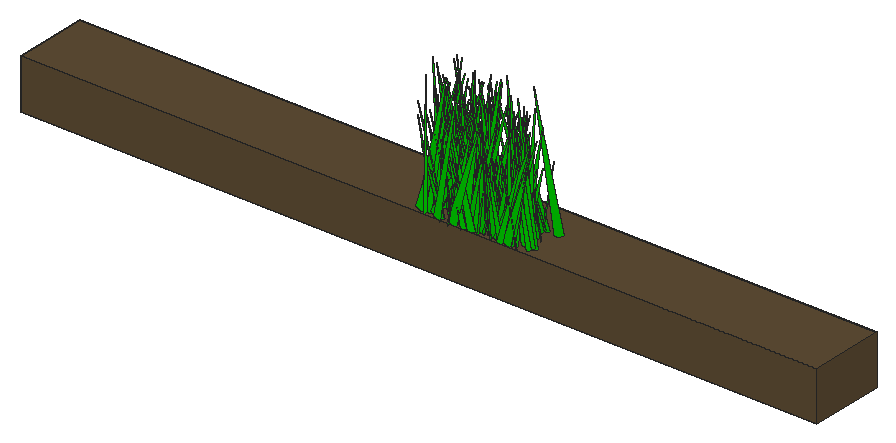
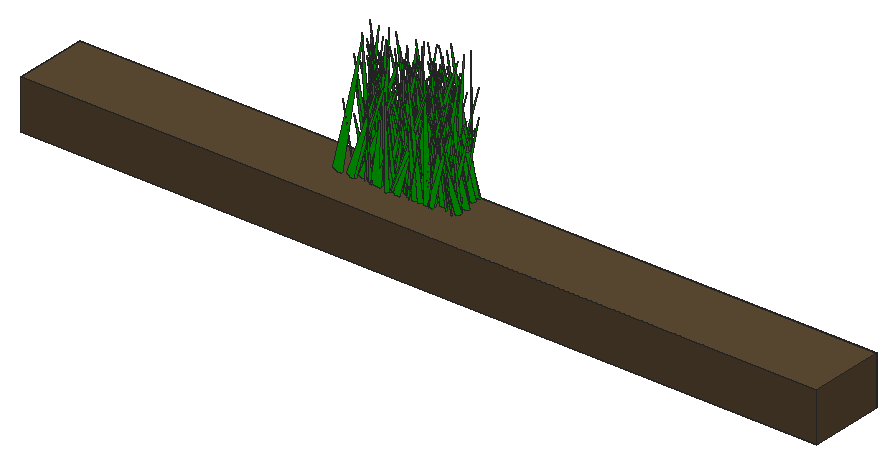
# SketchUp Ruby script. Lengths in inches.
U = 1.inch
M = Sketchup.active_model
def pt(a) = Geom::Point3d.new(a.map { |v| v * U })
def face(e, loops, mat)
  f = e.add_face(loops[0].map { |a| pt(a) })
  loops[1..].each { |l| e.add_face(l.map { |a| pt(a) }).erase! }
  f.material = f.back_material = mat if mat
  f
end
# faces: each face lists its corners as indices into pts; further lists are holes
def faces(e, pts, list, mat = nil) = list.each { |f| face(e, (f[0].is_a?(Array) ? f : [f]).map { |l| l.map { |i| pts[i] } }, mat) }
# xy, xz, yz: faces in a plane at the given z, y or x. An outline is a flat list of corners, or four numbers for a rectangle; further outlines are holes
def ring(l) = l.size == 4 ? [[l[0], l[1]], [l[2], l[1]], [l[2], l[3]], [l[0], l[3]]] : l.each_slice(2).to_a
def flat(e, list, mat, &to3) = list.each { |f| face(e, (f[0].is_a?(Array) ? f : [f]).map { |l| ring(l).map { |u, v| to3.(u, v) } }, mat) }
def xy(e, z, list, mat = nil) = flat(e, list, mat) { |x, y| [x, y, z] }
def xz(e, y, list, mat = nil) = flat(e, list, mat) { |x, z| [x, y, z] }
def yz(e, x, list, mat = nil) = flat(e, list, mat) { |y, z| [x, y, z] }
def lines(e, pts, list) = list.each { |a, b| e.add_line(pt(pts[a]), pt(pts[b])) }
# prism: a flat outline (further loops are holes) pulled along v
def prism(e, loops, v, mat = nil)
  f = face(e, loops, mat); d = Geom::Vector3d.new(v.map { |x| x * U })
  f.pushpull(f.normal.samedirection?(d) ? d.length : -d.length)
end
def box(e, o, s, mat = nil) = prism(e, [[o, [o[0] + s[0], o[1], o[2]], [o[0] + s[0], o[1] + s[1], o[2]], [o[0], o[1] + s[1], o[2]]]], [0, 0, s[2]], mat)
def at(x, y, z, deg = 0) = Geom::Transformation.translation(pt([x, y, z])) * Geom::Transformation.rotation(ORIGIN, Z_AXIS, deg.degrees)
def axes(o, x, y, z) = Geom::Transformation.new([*x, 0, *y, 0, *z, 0, *pt(o).to_a, 1])
def part(name) = M.definitions.add(name)
# library, detail: a bought-in or finely detailed component or shape, given as its bounding box
def library(name, o, s) = part(name).tap { |d| box(d.entities, o, s) }
def detail(e, o, s) = box(e.add_group.entities, o, s)
def put(e, d, t, mat = nil) = e.add_instance(d, t).tap { |i| i.material = mat if mat }
def group(e, t, mat = nil) = e.add_group.tap { |g| g.transformation = t; g.material = mat if mat }.entities
root = M.entities
M.materials.add("SOIL").color = [94, 77, 53]
M.materials.add("[Color G06]").color = [0, 204, 0]
c1 = part("fur_instance\#9")
p = [[0.8125,0,1.79],[0.67,-0.02,1.48],[0,-0.11,0],[0,0.11,0]]
faces(c1.entities,p,[[0,1,2,3]])
c2 = part("SOIL")
box(c2.entities,[0,0,0],[23.62,15.75,0.98],"SOIL")
put(root,c1,axes([64.27,19.94,4.28],[3.9337,-0.10201,2.1744],[-1.23525,-0.53254,2.12165],[-1.06111,0.24176,5.59098]),"[Color G06]")
put(root,c1,axes([66.12,17.16,4.28],[-3.59568,-0.13871,1.08691],[-1.16064,0.48631,-1.44733],[0.41383,0.15871,5.38474]),"[Color G06]")
put(root,c1,axes([66.23,19.01,4.28],[-2.06778,0.38398,1.15766],[2.83464,0.2572,1.51011],[-0.3835,-0.16929,4.92009]),"[Color G06]")
put(root,c1,axes([65.64,18.91,4.28],[-2.34714,-0.24884,0.13469],[-1.68843,0.31567,1.2736],[0.58467,-0.08736,4.21868]),"[Color G06]")
put(root,c2,axes([12.21,15.88,-2.33],[4.48996,0,0],[0,0.6261,0],[0,0,6.71057]),"[Color G06]")
put(root,c1,axes([65.53,16.66,4.28],[-4.03008,-0.15258,2.55922],[-0.6332,0.59823,1.86996],[1.93093,-0.12229,5.9546]),"[Color G06]")
put(root,c1,axes([64.93,20.74,4.28],[5.56804,0.19263,1.94531],[1.18681,-0.79236,1.42534],[-1.48118,0.08926,8.45483]),"[Color G06]")
put(root,c1,axes([65.28,18.91,4.28],[-4.27988,-0.612,0.13864],[-3.47082,0.48283,5.50199],[2.68766,-0.35103,7.32598]),"[Color G06]")
put(root,c1,axes([66.875,19.08,4.28],[0.00173,-0.4781,0.37924],[-3.2834,-0.01072,-1.51908],[-1.0193,0.03372,4.89395]),"[Color G06]")
put(root,c1,axes([64.82,18.02,4.28],[4.41749,0.02868,0.97094],[-0.02479,-0.58705,2.24414],[-0.68098,0.20744,6.21676]),"[Color G06]")
put(root,c1,axes([66.66,18.07,4.28],[2.23144,-0.72846,3.30583],[-5.41989,-0.37165,-1.23578],[-1.6756,0.23202,8.39972]),"[Color G06]")
put(root,c1,axes([66.01,18.3,4.28],[2.74843,0.58472,1.17107],[4.10613,-0.39786,1.29411],[-1.15604,-0.02302,7.38067]),"[Color G06]")
put(root,c1,axes([65.93,16.13,4.28],[5.28818,-0.28174,2.69175],[-1.63303,-0.7717,-2.11244],[-2.15849,-0.10641,8.19284]),"[Color G06]")
put(root,c1,axes([67.66,19.3,4.28],[-4.5157,0.45036,1.85261],[3.42037,0.6238,1.20327],[0.5177,-0.19305,8.2098]),"[Color G06]")
put(root,c1,axes([64.86,18.26,4.28],[1.2715,-0.352,0.82952],[-2.32783,-0.11849,2.1945],[1.12305,0.15293,3.60956]),"[Color G06]")
put(root,c1,axes([64.29,20.21,4.28],[2.89965,-0.47126,0.48649],[-3.21633,-0.36216,2.52086],[1.08732,0.18544,6.15941]),"[Color G06]")
put(root,c1,axes([67.61,20.84,4.28],[0.74196,-0.52967,0.07225],[-3.46204,-0.09711,-2.36776],[-1.56343,-0.03632,5.27742]),"[Color G06]")
put(root,c1,axes([65.63,18.85,4.28],[1.34326,0.36408,0.84996],[2.64038,-0.1672,-1.09373],[0.41087,-0.11584,4.24991]),"[Color G06]")
put(root,c1,axes([68.07,16.52,4.28],[-4.76111,-0.23036,0.10058],[-1.58818,0.64517,1.81412],[0.45963,-0.15694,7.31027]),"[Color G06]")
put(root,c1,axes([64.39,18.875,4.28],[3.81948,0.65894,0.41305],[4.68317,-0.51885,-1.64937],[0.68832,-0.12631,8.93]),"[Color G06]")
put(root,c1,axes([66.84,17.08,4.28],[-3.36168,0.48783,1.26493],[3.33459,0.4829,-1.59837],[1.35477,0.02188,7.07294]),"[Color G06]")
put(root,c1,axes([65.9,18.96,4.28],[-4.17835,0.54975,0.89849],[2.79534,0.49034,-5.42673],[2.84426,0.3257,6.65331]),"[Color G06]")
put(root,c1,axes([67.83,20.375,4.28],[-0.79878,-0.71008,0.86951],[-5.06087,0.0963,-1.35143],[-0.81022,0.09857,7.58425]),"[Color G06]")
put(root,c1,axes([68.07,16.24,4.28],[-1.79719,-0.34848,0.05868],[-2.42683,0.24169,-1.14114],[-0.59772,0.06647,4.45677]),"[Color G06]")
put(root,c1,axes([64.9375,16.33,4.28],[2.13707,0.68454,1.01733],[4.81023,-0.26161,-2.34953],[1.19326,-0.1714,7.64932]),"[Color G06]")
put(root,c1,axes([65.19,16.55,4.28],[-1.2259,-0.82669,2.42771],[-5.62709,0.24389,3.1931],[2.47397,0.14508,8.46575]),"[Color G06]")
put(root,c1,axes([66.25,18.01,4.28],[3.08494,0.15001,0.2605],[0.88845,-0.38846,2.19393],[-0.63105,0.18641,4.36231]),"[Color G06]")
put(root,c1,axes([66.37,19.62,4.28],[-1.44395,0.338,1.23713],[2.15076,0.23196,-1.67262],[1.39086,-0.00779,3.87082]),"[Color G06]")
put(root,c1,axes([65.86,20.33,4.28],[5.05978,0.1564,1.77856],[1.34323,-0.70526,-1.41146],[-0.93265,-0.16723,7.61609]),"[Color G06]")
put(root,c1,axes([64.8125,17.16,4.28],[5.71437,-0.35675,0.81278],[-2.61535,-0.7814,1.67358],[-0.02906,0.17354,9.20654]),"[Color G06]")
put(root,c1,axes([66.28,19.2,4.28],[4.30909,-0.14199,2.05065],[-1.42182,-0.58584,2.01409],[-0.94751,0.23337,6.30366]),"[Color G06]")
put(root,c1,axes([69.3125,19.57,4.28],[-5.52745,0.03843,0.24282],[0.22598,0.74656,-2.08225],[0.22645,0.19303,8.00506]),"[Color G06]")
put(root,c1,axes([67.84,20.68,4.28],[-3.57294,0.06411,1.38728],[0.20503,0.49942,-1.47175],[1.01534,0.12475,5.17899]),"[Color G06]")
put(root,c1,axes([66.63,19.9,4.28],[-1.10752,-0.6635,1.1429],[-4.62289,0.17718,1.80941],[1.36144,0.06188,7.07373]),"[Color G06]")
put(root,c1,axes([67.22,18.42,4.28],[4.87658,0.467,1.34273],[2.8491,-0.66289,3.37128],[-1.97624,0.1967,8.17365]),"[Color G06]")
put(root,c1,axes([66.07,16.44,4.28],[4.96611,-0.36753,1.97979],[-2.87532,-0.6839,1.52607],[-0.65883,0.21437,8.26304]),"[Color G06]")
put(root,c1,axes([66.57,17.35,4.28],[-0.59285,0.44163,1.9606],[3.16914,0.14138,-1.51769],[1.30675,-0.14251,4.57019]),"[Color G06]")
put(root,c1,axes([68.84,17.19,4.28],[-4.91803,-0.20416,0.17663],[-1.24803,0.61118,3.52939],[0.77451,-0.31152,6.80875]),"[Color G06]")
put(root,c1,axes([68.7,20.35,4.28],[-5.8108,0.01733,2.20475],[-0.05639,0.83002,-1.08167],[1.47933,0.09973,8.61904]),"[Color G06]")
put(root,c1,axes([68,17.33,4.28],[-2.34423,-0.18821,0.49656],[-1.15107,0.31378,1.5235],[0.77914,-0.1027,3.74478]),"[Color G06]")
put(root,c1,axes([69.53,20.3,4.28],[-2.66158,0.52184,0.92971],[3.72924,0.34047,1.89447],[-0.69586,-0.17132,6.59678]),"[Color G06]")
put(root,c1,axes([66.15,18.34,4.28],[4.53169,0.0066,0.17546],[0.00744,-0.59921,2.15905],[-0.12635,0.20134,6.41998]),"[Color G06]")
put(root,c1,axes([69.43,16.26,4.28],[-5.68691,0.08802,1.10084],[0.3155,0.74548,-3.20639],[0.91727,0.28928,7.92784]),"[Color G06]")
put(root,c1,axes([70.48,17.39,4.28],[-1.74227,-0.51191,0.57615],[-3.12279,0.17272,-3.46489],[-1.96806,0.17912,4.98781]),"[Color G06]")
put(root,c1,axes([65.21,19.46,4.28],[5.78095,-0.27577,0.1135],[-1.90726,-0.76757,2.75583],[0.52838,0.24657,8.70587]),"[Color G06]")
put(root,c1,axes([67.34,16.21,4.28],[-0.97561,0.32933,1.80319],[2.35163,0.1903,-1.15043],[1.22598,-0.10295,3.64164]),"[Color G06]")
put(root,c1,axes([67.75,19.18,4.28],[3.09749,-0.22392,0.88391],[-1.41414,-0.43098,-1.47269],[-0.96366,-0.08731,5.00229]),"[Color G06]")
put(root,c1,axes([68,19.7,4.28],[2.92193,-0.21443,1.09605],[-1.31963,-0.41328,-1.42956],[-1.07745,-0.07533,4.72326]),"[Color G06]")
put(root,c1,axes([66.02,17.58,4.28],[2.45604,-0.70792,0.71225],[-4.85278,-0.30188,2.91186],[1.56531,0.17488,7.90979]),"[Color G06]")
put(root,c1,axes([68,20.78,4.28],[-1.27431,-0.73556,1.5677],[-5.26886,0.20089,1.26122],[1.07877,0.1123,8.01183]),"[Color G06]")
put(root,c1,axes([65.85,19.25,4.28],[3.02053,-0.58933,0.27626],[-3.90663,-0.37645,3.15948],[1.62277,0.19067,7.09185]),"[Color G06]")
put(root,c1,axes([68.76,18.32,4.28],[3.35805,0.30855,1.56651],[1.83431,-0.48137,2.10828],[-1.62168,0.09443,5.62853]),"[Color G06]")
put(root,c1,axes([66.32,18.14,4.28],[5.01438,0.22789,0.47335],[1.61835,-0.63452,-3.20234],[0.39,-0.29709,7.20253]),"[Color G06]")
put(root,c1,axes([70.48,19.6,4.28],[-3.13704,-0.74976,1.17592],[-5.41814,0.42191,-1.38487],[-0.41462,0.15934,9.20002]),"[Color G06]")
put(root,c1,axes([67.78,19.27,4.28],[-1.94172,-0.3878,3.30736],[-2.88964,0.37698,1.28819],[2.06906,0.16255,4.90289]),"[Color G06]")
put(root,c1,axes([67.59,15.91,4.28],[3.54088,0.51335,2.57501],[4.06154,-0.45916,-1.96012],[-0.15678,-0.30115,7.37812]),"[Color G06]")
put(root,c1,axes([69.05,17.05,4.28],[-3.17062,0.45416,0.91994],[3.06388,0.4469,-1.7563],[1.26446,0.05594,6.5624]),"[Color G06]")
put(root,c1,axes([68.75,17.77,4.28],[4.24094,-0.29055,3.7921],[-2.78852,-0.62384,1.47521],[-1.73297,0.29279,6.90627]),"[Color G06]")
put(root,c1,axes([71.55,17.78,4.28],[-5.17247,-0.46056,0.00062],[-3.27844,0.71595,-1.11271],[-0.40033,0.08753,9.10447]),"[Color G06]")
put(root,c1,axes([68.38,18.43,4.28],[-1.87229,-0.7605,1.04521],[-5.23346,0.27808,2.30206],[1.68632,0.01863,8.30486]),"[Color G06]")
put(root,c1,axes([66.77,16.4,4.28],[2.33579,0.49121,0.1582],[3.08444,-0.27637,-3.14717],[1.7048,-0.17299,5.47731]),"[Color G06]")
put(root,c1,axes([69.96,17.8,4.28],[0.9333,-0.63025,1.21187],[-4.43375,-0.1537,-1.55525],[-1.19446,0.07809,6.71987]),"[Color G06]")
put(root,c1,axes([68.34,19.38,4.28],[3.11376,0.25616,0.9973],[1.94448,-0.42367,-1.06016],[-0.19703,-0.13299,5.29824]),"[Color G06]")
put(root,c1,axes([68.78,19.79,4.28],[-1.77394,0.70053,1.87694],[4.92633,0.28534,-1.83386],[1.59562,-0.10216,7.74859]),"[Color G06]")
put(root,c1,axes([68.23,18.93,4.28],[0.76642,0.55479,0.85726],[3.87739,-0.08056,-1.75415],[1.06014,-0.10644,5.79597]),"[Color G06]")
put(root,c1,axes([68.67,18.69,4.28],[0.09815,0.48947,2.17089],[3.68366,0.03723,-1.33642],[0.92802,-0.19956,5.07514]),"[Color G06]")
put(root,c1,axes([70.64,17.76,4.28],[-2.64218,-0.5957,2.25383],[-4.53026,0.34741,-1.31518],[-0.00041,0.24347,7.3911]),"[Color G06]")
put(root,c1,axes([68.59,18.15,4.28],[-0.66244,0.63721,1.68644],[4.49181,0.13307,-1.83449],[1.40654,-0.12484,6.65274]),"[Color G06]")
put(root,c1,axes([70.63,20.5625,4.28],[-3.75467,0.03192,0.77655],[0.07252,0.50757,-1.61376],[0.56313,0.14749,5.38546]),"[Color G06]")
put(root,c1,axes([69.33,15.95,4.28],[3.14663,0.29996,0.76242],[1.92015,-0.43215,1.82907],[-1.09564,0.10412,5.39514]),"[Color G06]")
put(root,c1,axes([68.43,18.98,4.28],[3.89803,-0.05532,0.69047],[-0.52017,-0.51951,1.7781],[-0.31662,0.1724,5.57952]),"[Color G06]")
put(root,c1,axes([70.31,19.58,4.28],[-3.14948,-0.17379,0.85258],[-0.96371,0.42253,1.94177],[0.97463,-0.1438,4.67506]),"[Color G06]")
put(root,c1,axes([71.11,15.96,4.28],[-2.60426,0.31734,0.66766],[2.31494,0.35007,1.05631],[-0.13964,-0.11495,5.05986]),"[Color G06]")
put(root,c1,axes([69,20.73,4.28],[4.80759,-0.32738,2.5492],[-2.66959,-0.67939,1.22332],[-1.13763,0.21079,7.90214]),"[Color G06]")
put(root,c1,axes([68.38,19.17,4.28],[4.77946,-0.11552,0.35589],[-0.76083,-0.65332,-1.53635],[-0.40506,-0.13587,7.0851]),"[Color G06]")
put(root,c1,axes([68.74,18.33,4.28],[3.73699,0.09804,0.06654],[0.64732,-0.49107,1.91444],[-0.27806,0.17447,5.35104]),"[Color G06]")
put(root,c1,axes([69.74,20.74,4.28],[-0.83593,0.48498,0.0355],[3.40191,0.11472,-1.10362],[0.72342,0.02091,5.23086]),"[Color G06]")
put(root,c1,axes([72.08,16.22,4.28],[-2.79763,-0.54176,1.73604],[-3.93774,0.31597,-2.84743],[-0.9682,0.28033,6.56439]),"[Color G06]")
put(root,c1,axes([70.22,17.8,4.28],[3.52732,0.2393,1.90503],[1.22279,-0.50717,2.26093],[-1.75339,0.12771,5.40912]),"[Color G06]")
put(root,c1,axes([68.68,18.1875,4.28],[-0.38735,-0.50805,1.24588],[-3.30073,0.10132,2.45407],[1.7533,0.07851,4.89525]),"[Color G06]")
put(root,c1,axes([72.33,20.92,4.28],[-0.69251,-0.73769,0.90073],[-4.94749,0.05784,-3.05542],[-1.96768,0.11421,7.36545]),"[Color G06]")
put(root,c1,axes([71.04,20.35,4.28],[-4.47876,0.12906,1.72291],[0.69894,0.63677,-1.42098],[1.30269,0.10208,6.68593]),"[Color G06]")
put(root,c1,axes([72.41,20.88,4.28],[-4.00422,0.36649,1.21006],[2.71666,0.49613,2.81914],[-0.42755,-0.27996,6.58009]),"[Color G06]")
put(root,c1,axes([70.42,19.05,4.28],[5.14472,0.18763,4.15161],[2.00102,-0.77602,-1.51019],[-2.34999,-0.25002,7.80299]),"[Color G06]")
put(root,c1,axes([69.62,17.22,4.28],[0.89904,-0.44398,1.50676],[-3.30658,-0.09789,1.09364],[0.469,0.16093,4.82214]),"[Color G06]")
put(root,c1,axes([71.74,19.78,4.28],[1.93246,-0.63051,2.31923],[-4.19713,-0.33551,-2.66608],[-2.28835,0.08291,6.84847]),"[Color G06]")
put(root,c1,axes([72.15,15.93,4.28],[-2.93158,0.54127,0.79353],[3.88045,0.38844,1.58535],[-0.5392,-0.14733,7.09501]),"[Color G06]")
put(root,c1,axes([68.92,20.06,4.28],[-0.8905,0.7007,0.485],[4.53534,0.13158,-3.23612],[2.18761,0.01245,6.90653]),"[Color G06]")
put(root,c1,axes([71.4,17.24,4.28],[-4.46899,-0.31452,0.96618],[-2.08366,0.62115,1.69961],[1.07867,-0.10319,7.28608]),"[Color G06]")
put(root,c1,axes([70.82,18.35,4.28],[-3.7058,0.36945,1.50512],[2.47006,0.53432,-1.48184],[1.39014,0.03547,6.6453]),"[Color G06]")
put(root,c1,axes([69.46,17.3,4.28],[-0.436,-0.63405,1.0117],[-4.36584,0.0868,2.04652],[1.43957,0.07122,6.51295]),"[Color G06]")
put(root,c1,axes([71.59,18.21,4.28],[2.44043,-0.72747,0.0396],[-4.71253,-0.30915,-3.67601],[-2.23804,-0.1423,7.78359]),"[Color G06]")
put(root,c1,axes([69.5,16.21,4.28],[2.98468,-0.35426,1.75326],[-2.79624,-0.38664,1.6587],[-0.10587,0.2247,5.61822]),"[Color G06]")
put(root,c1,axes([69.09,16.14,4.28],[6.01942,-0.14511,0.93493],[-0.70864,-0.7781,-3.68203],[-0.98593,-0.32669,8.35452]),"[Color G06]")
put(root,c1,axes([71.75,16.86,4.28],[0.53293,0.76061,0.64122],[5.27361,-0.08742,2.12228],[-1.45788,-0.0382,7.91136]),"[Color G06]")
put(root,c1,axes([69.25,17.06,4.28],[5.06302,-0.16125,0.57283],[-1.08501,-0.70076,-1.23853],[-0.55387,-0.10121,7.66246]),"[Color G06]")
put(root,c1,axes([68.96,20.27,4.28],[3.98403,-0.42734,0.58357],[-3.07576,-0.54037,1.4485],[0.289,0.14002,7.37123]),"[Color G06]")
put(root,c1,axes([72.46,18.84,4.28],[-0.86922,-0.46107,1.86134],[-3.26388,0.03629,-2.37197],[-1.35312,0.20865,4.52578]),"[Color G06]")
put(root,c1,axes([70.02,16.68,4.28],[2.6038,-0.32471,1.03628],[-2.42963,-0.34818,1.1038],[-0.00322,0.14126,5.10276]),"[Color G06]")
put(root,c1,axes([72.77,16.8,4.28],[-4.81253,0.11411,0.86308],[0.96009,0.63818,2.26529],[0.28531,-0.22265,6.93535]),"[Color G06]")
put(root,c1,axes([70.08,19.58,4.28],[5.74229,-0.26623,1.55376],[-1.63196,-0.79842,-2.24328],[-1.43617,-0.15721,8.76158]),"[Color G06]")
put(root,c1,axes([70.27,18.27,4.28],[4.77431,0.01175,1.798],[-0.1042,-0.6784,1.12749],[-1.20146,0.10554,7.04704]),"[Color G06]")
put(root,c1,axes([70.24,20.01,4.28],[2.1619,-0.21323,1.09014],[-1.69157,-0.26253,1.5946],[0.09403,0.17974,3.62221]),"[Color G06]")
put(root,c1,axes([71.96,18.06,4.28],[-4.37224,0.04611,1.70218],[0.01924,0.60934,-1.78582],[1.18578,0.16013,6.30528]),"[Color G06]")
put(root,c1,axes([71.87,18.24,4.28],[-5.5981,0.1309,3.0974],[1.28319,0.81549,1.22145],[1.87872,-0.16694,8.39519]),"[Color G06]")
put(root,c1,axes([72.88,16.91,4.28],[-5.37867,-0.33174,2.04235],[-2.65038,0.73664,-1.84638],[0.70882,0.2371,8.59392]),"[Color G06]")
put(root,c1,axes([72.2,18.17,4.28],[-2.68769,-0.10307,0.12403],[-0.6596,0.35034,1.51666],[0.34373,-0.13364,3.88021]),"[Color G06]")
put(root,c1,axes([72.72,17.43,4.28],[-1.54656,0.35333,0.37365],[2.45565,0.19621,1.38967],[-0.67277,-0.09605,4.21344]),"[Color G06]")
put(root,c1,axes([69.59,15.95,4.28],[1.56377,-0.64305,1.71527],[-4.51442,-0.1484,2.80235],[1.48421,0.22614,6.71652]),"[Color G06]")
put(root,c1,axes([71.07,20.49,4.28],[4.30544,-0.46371,0.68313],[-3.06103,-0.58494,-2.51783],[-1.37736,-0.14953,7.73098]),"[Color G06]")
put(root,c1,axes([71.68,18.2,4.28],[2.67697,-0.02127,2.0865],[-0.69009,-0.38488,1.52707],[-1.22311,0.17061,3.70505]),"[Color G06]")
put(root,c1,axes([71.69,20.05,4.28],[2.87234,0.53611,0.9293],[3.68948,-0.40908,1.63697],[-1.2471,0.02455,6.98329]),"[Color G06]")
put(root,c1,axes([73.04,20.51,4.28],[-5.20772,-0.06627,1.64039],[-0.77294,0.70826,-2.19436],[0.91272,0.22168,7.5013]),"[Color G06]")
put(root,c1,axes([70.79,18.91,4.28],[4.47878,0.56246,0.84443],[3.96382,-0.62886,1.15652],[-0.93647,0.02824,8.93379]),"[Color G06]")
put(root,c1,axes([74.08,16.76,4.28],[-4.85543,0.19551,0.29225],[1.3739,0.62735,2.77653],[-0.34105,-0.25611,7.02444]),"[Color G06]")
put(root,c1,axes([72.96,18.99,4.28],[-4.00508,0.18925,0.23189],[1.24887,0.53446,-1.92391],[0.55337,0.16351,6.02026]),"[Color G06]")
put(root,c1,axes([70.82,16.37,4.28],[-1.77059,0.64114,4.01565],[4.89711,0.35114,-1.61709],[2.09207,-0.27934,7.18388]),"[Color G06]")
put(root,c1,axes([70.95,20.42,4.28],[5.85885,-0.26036,1.26138],[-1.4984,-0.78757,-3.1281],[-1.39758,-0.24708,8.64165]),"[Color G06]")
put(root,c1,axes([74.1,19.61,4.28],[-1.18591,0.74302,2.67414],[5.36757,0.07403,2.95428],[-1.66814,-0.29003,7.60491]),"[Color G06]")
put(root,c1,axes([71.1,19.44,4.28],[1.17388,-0.60655,1.3276],[-4.38323,-0.13802,1.4136],[0.70445,0.15195,6.58348]),"[Color G06]")
put(root,c1,axes([73.39,19.82,4.28],[-0.43736,0.47588,0.91151],[3.35739,0.03678,1.39245],[-0.86389,-0.09798,4.95011]),"[Color G06]")
put(root,c1,axes([71.33,18.2,4.28],[2.2843,0.7886,2.01921],[5.79368,-0.29165,-1.55606],[0.49019,-0.22781,8.98185]),"[Color G06]")
put(root,c1,axes([73.54,19.61,4.28],[-4.80021,-0.12629,1.59289],[-0.66645,0.67363,1.64907],[1.22962,-0.12791,7.11217]),"[Color G06]")
put(root,c1,axes([71.51,16.39,4.28],[3.64774,0.3296,2.29646],[2.81376,-0.44731,-2.6087],[-0.17424,-0.32336,5.94947]),"[Color G06]")
put(root,c1,axes([72.59,16.66,4.28],[-2.50037,-0.52412,1.72298],[-3.64478,0.38045,1.4795],[1.47363,0.05168,6.58273]),"[Color G06]")
put(root,c1,axes([73.95,18.89,4.28],[-5.59903,0.27073,1.38164],[1.59173,0.76355,-2.77882],[1.44581,0.20782,8.40977]),"[Color G06]")
put(root,c1,axes([72.49,20.66,4.28],[-0.71622,-0.40597,1.3613],[-2.87436,0.1335,1.19542],[1.02144,0.09102,4.31849]),"[Color G06]")
put(root,c1,axes([72.15,19.33,4.28],[-0.53569,0.51917,1.20271],[3.55225,0.109,-1.87067],[1.37499,-0.07932,5.30139]),"[Color G06]")
put(root,c1,axes([74.52,17.27,4.28],[0.32405,0.79012,2.01937],[5.6187,-0.09217,2.12898],[-1.53657,-0.17042,8.2108]),"[Color G06]")
put(root,c1,axes([73.59,17.43,4.28],[-4.93081,0.2989,2.28793],[1.79653,0.71295,-2.05096],[1.92624,0.10018,7.76952]),"[Color G06]")
put(root,c1,axes([73.17,16.46,4.28],[-2.49454,-0.55736,1.11301],[-3.85108,0.36298,1.6003],[1.3036,0.00576,6.85745]),"[Color G06]")
put(root,c1,axes([71.51,18.08,4.28],[3.49204,0.56909,1.79571],[4.22695,-0.43958,-2.3579],[0.48166,-0.26825,7.67357]),"[Color G06]")
put(root,c1,axes([72.0625,16.41,4.28],[1.21017,0.65067,0.5218],[4.58555,-0.15491,-1.56602],[0.93135,-0.08278,7.03235]),"[Color G06]")
put(root,c1,axes([73.08,21.23,4.28],[-2.82563,-0.43908,1.15691],[-2.80084,0.40265,2.27443],[1.63381,-0.06912,5.8999]),"[Color G06]")
put(root,c1,axes([73.13,15.9,4.28],[3.9495,0.26929,0.70307],[1.32887,-0.46626,3.84049],[-1.47808,0.30036,5.33143]),"[Color G06]")
put(root,c1,axes([72.71,16.82,4.28],[3.16276,-0.23114,0.02791],[-1.58923,-0.42439,-1.46662],[-0.47143,-0.12004,5.13134]),"[Color G06]")
put(root,c1,axes([74.37,17.72,4.28],[-4.4443,-0.037,1.82671],[-0.47252,0.6322,-1.09697],[1.158,0.11596,6.56311]),"[Color G06]")
put(root,c1,axes([75.03,16.5,4.28],[-2.1333,-0.68445,0.89669],[-4.91148,0.28271,-1.31167],[-0.57402,0.12478,7.89058]),"[Color G06]")
put(root,c1,axes([71.11,18.63,4.28],[5.01665,-0.36755,0.02338],[-2.56063,-0.67845,2.0525],[0.62532,0.17051,8.21722]),"[Color G06]")
put(root,c1,axes([72.86,19.21,4.28],[0.28567,0.64465,1.30007],[4.61138,-0.01437,-1.44466],[0.92916,-0.12686,6.77008]),"[Color G06]")
put(root,c1,axes([74.18,16.78,4.28],[1.0824,0.43036,0.08378],[2.96044,-0.14708,1.35555],[-0.87382,0.03478,4.69629]),"[Color G06]")
put(root,c1,axes([74.23,16.47,4.28],[-3.05765,-0.22895,0.72092],[-1.42019,0.41635,1.73399],[0.95465,-0.11391,4.8886]),"[Color G06]")
put(root,c1,axes([75.125,17.75,4.28],[-5.24145,0.37213,0.2626],[2.4037,0.67913,-3.38457],[1.17244,0.27128,8.11294]),"[Color G06]")
put(root,c1,axes([74.93,20.78,4.28],[1.16518,-0.76521,2.8333],[-5.61812,-0.2166,-1.55907],[-1.46397,0.22218,8.2381]),"[Color G06]")
put(root,c1,axes([74.42,20.57,4.28],[-3.02768,0.34403,0.30976],[2.23464,0.39939,-2.16558],[1.06578,0.1399,5.42057]),"[Color G06]")
put(root,c1,axes([72.91,20.9,4.28],[-1.11881,-0.62216,0.02903],[-4.03447,0.14226,2.9291],[1.90526,-0.0641,6.21955]),"[Color G06]")
put(root,c1,axes([73.33,19.28,4.28],[4.10029,0.06396,1.54491],[0.77369,-0.55406,-1.95177],[-0.82479,-0.20177,5.84937]),"[Color G06]")
put(root,c1,axes([74.65,15.96,4.28],[-3.41823,-0.16721,1.36846],[-0.93217,0.4827,1.57417],[1.18628,-0.10251,5.18012]),"[Color G06]")
put(root,c1,axes([73.61,17.06,4.28],[-2.05688,0.38937,1.43078],[2.39097,0.31518,-2.17527],[1.73101,0.02732,4.70473]),"[Color G06]")
put(root,c1,axes([72.375,18.34,4.28],[3.31039,-0.56284,0.81716],[-4.0134,-0.43397,1.98088],[0.69504,0.17486,7.54628]),"[Color G06]")
put(root,c1,axes([76.34,17.72,4.28],[-4.03019,0.25606,0.43563],[1.82878,0.52845,2.1102],[-0.33528,-0.19552,6.27379]),"[Color G06]")
put(root,c1,axes([72.93,19.4375,4.28],[3.20471,0.1635,0.27258],[1.16866,-0.42219,-1.59994],[0.20572,-0.14869,4.84275]),"[Color G06]")
put(root,c1,axes([73.52,16.32,4.28],[3.44273,0.07247,1.14582],[0.76194,-0.45555,-1.80418],[-0.52656,-0.1854,4.88093]),"[Color G06]")
put(root,c1,axes([77.22,20.27,4.28],[-3.2478,0.49746,0.11157],[3.39776,0.42687,2.29823],[-1.08957,-0.15167,6.8343]),"[Color G06]")
put(root,c1,axes([76.03,15.98,4.28],[-1.14046,0.39552,0.91868],[2.85011,0.13526,1.21394],[-0.54762,-0.11977,4.40484]),"[Color G06]")
put(root,c1,axes([75.52,17.2,4.28],[-2.52658,-0.17387,0.06484],[-1.04952,0.30358,2.16535],[0.67461,-0.17889,3.61157]),"[Color G06]")
put(root,c1,axes([74.61,18.49,4.28],[-0.91561,-0.63845,0.04836],[-4.46381,0.1255,1.54322],[1.01871,-0.02392,6.80556]),"[Color G06]")
put(root,c1,axes([75.375,19.95,4.28],[-2.82828,-0.33019,1.01645],[-2.11188,0.3993,1.77421],[1.26862,-0.07142,5.21965]),"[Color G06]")
put(root,c1,axes([77.12,17.27,4.28],[-1.42085,0.40596,0.51594],[2.68035,0.15822,2.18717],[-1.1875,-0.12861,4.31942]),"[Color G06]")
put(root,c1,axes([77.6875,18.71,4.28],[-2.64589,0.50951,0.77284],[3.49882,0.31816,2.66153],[-1.17313,-0.20026,6.19484]),"[Color G06]")
put(root,c1,axes([74.16,18.03,4.28],[0.66068,0.68795,1.28599],[4.83382,-0.05597,-2.10776],[1.309,-0.14054,7.13439]),"[Color G06]")
put(root,c1,axes([78.45,19.09,4.28],[-4.07955,-0.60152,1.18407],[-4.19722,0.49168,-3.60837],[-1.27234,0.30671,8.10683]),"[Color G06]")
put(root,c1,axes([75.62,20.77,4.28],[2.13387,0.28604,0.18207],[1.83022,-0.27569,1.84111],[-0.93428,0.11324,4.02251]),"[Color G06]")
put(root,c1,axes([74.97,20.07,4.28],[-0.09874,0.55012,1.39939],[3.953,0.04212,-1.27899],[0.90211,-0.12435,5.75765]),"[Color G06]")
put(root,c1,axes([76.02,19.66,4.28],[-3.05111,0.30829,0.39383],[1.93953,0.39864,-2.2824],[1.09329,0.15315,5.1481]),"[Color G06]")
put(root,c1,axes([78.17,20.27,4.28],[-4.98506,-0.27671,0.7298],[-1.99994,0.62368,-3.34969],[-0.42013,0.31445,7.28603]),"[Color G06]")
put(root,c1,axes([75.59,18.66,4.28],[-4.45112,-0.43476,1.70508],[-2.34081,0.59967,3.91511],[2.35432,-0.22574,7.11629]),"[Color G06]")
put(root,c1,axes([74.91,16.69,4.28],[-0.88008,-0.4473,2.08809],[-3.12414,0.19091,1.75667],[1.57521,0.12872,4.65066]),"[Color G06]")
put(root,c1,axes([76.71,18.03,4.28],[0.17546,0.81297,0.98222],[5.80961,-0.03686,1.18645],[-0.81809,-0.0874,8.6362]),"[Color G06]")
put(root,c1,axes([76.13,20.48,4.28],[2.8076,-0.02836,2.09433],[0.49403,-0.38704,-2.08145],[-1.32699,-0.2041,3.65619]),"[Color G06]")
put(root,c1,axes([76.5625,20.49,4.28],[-3.84948,0.09174,1.60024],[0.12247,0.5062,-2.67567],[1.2507,0.2328,5.18733]),"[Color G06]")
put(root,c1,axes([75.66,18.25,4.28],[4.71657,-0.21034,1.60525],[-1.16267,-0.65538,-2.23397],[-1.44118,-0.15965,7.05576]),"[Color G06]")
put(root,c1,axes([77.91,20.76,4.28],[-1.66109,-0.45378,0.90352],[-3.17018,0.19101,-1.99844],[-0.95136,0.1558,5.08176]),"[Color G06]")
put(root,c1,axes([78.35,20.88,4.28],[-2.51401,-0.566,0.60416],[-3.95649,0.32226,-2.09463],[-0.99225,0.14908,6.8214]),"[Color G06]")
put(root,c1,axes([76.89,16.92,4.28],[-5.42398,-0.07816,3.28802],[-1.07288,0.78847,-1.80045],[2.00073,0.21093,7.94834]),"[Color G06]")
put(root,c1,axes([74.82,17.72,4.28],[3.3823,-0.44761,0.9381],[-3.24513,-0.44355,1.82376],[0.40816,0.18269,6.72632]),"[Color G06]")
put(root,c1,axes([76.77,19.64,4.28],[4.60467,0.0584,3.65283],[1.01415,-0.7003,-1.56952],[-2.26281,-0.19502,6.72983]),"[Color G06]")
put(root,c1,axes([74.94,17.63,4.28],[5.48478,0.14499,0.58786],[0.9453,-0.75359,1.65079],[-0.58504,0.14169,8.17848]),"[Color G06]")
put(root,c1,axes([75.9,20.47,4.28],[1.36624,0.47123,1.80326],[3.56108,-0.15594,-1.34544],[0.4409,-0.20071,5.27908]),"[Color G06]")
put(root,c1,axes([77.77,19.375,4.28],[-4.29117,-0.07166,1.81916],[-0.77336,0.6039,-1.34211],[1.07123,0.14891,6.31832]),"[Color G06]")
put(root,c1,axes([75.92,18.95,4.28],[-0.17864,-0.43069,1.18755],[-2.88549,0.06909,1.90884],[1.35822,0.09013,4.21146]),"[Color G06]")
put(root,c1,axes([76.77,18.02,4.28],[3.48767,0.56497,1.09017],[3.94059,-0.49674,1.41238],[-1.19121,0.01089,7.86407]),"[Color G06]")
put(root,c1,axes([76.92,16.28,4.28],[3.55952,-0.47451,1.03586],[-3.19377,-0.50165,-1.88315],[-1.36357,-0.06369,7.11482]),"[Color G06]")
put(root,c1,axes([78.59,17.11,4.28],[-0.67065,0.73005,1.47962],[5.17589,0.05624,2.05286],[-1.26471,-0.15697,7.61682]),"[Color G06]")
put(root,c1,axes([76.51,20.15,4.28],[-1.55344,0.38989,0.25169],[2.35375,0.19626,-2.47307],[1.51843,0.09465,4.09104]),"[Color G06]")
put(root,c1,axes([75.39,18.4,4.28],[2.47224,-0.55425,0.34121],[-3.85435,-0.32382,1.95658],[0.99718,0.12249,6.71668]),"[Color G06]")
put(root,c1,axes([76.13,17.82,4.28],[1.05404,-0.58465,0.62019],[-4.12673,-0.13124,1.45379],[0.84911,0.0879,6.29561]),"[Color G06]")
put(root,c1,axes([78.09,16.03,4.28],[-3.79703,-0.19556,0.42051],[-1.12922,0.47815,2.76824],[0.87795,-0.23078,5.37913]),"[Color G06]")
put(root,c1,axes([75.99,15.91,4.28],[2.71552,-0.3878,0.6107],[-2.7908,-0.36252,1.27489],[0.33516,0.12333,5.66764]),"[Color G06]")
put(root,c1,axes([76.27,18.23,4.28],[-0.12404,0.48966,0.12197],[3.18952,0.02047,-2.19544],[1.47104,-0.0031,4.77046]),"[Color G06]")
put(root,c1,axes([78.15,17.36,4.28],[-3.96365,0.20983,2.32486],[1.84503,0.5642,1.17681],[1.13129,-0.18499,6.22626]),"[Color G06]")
put(root,c1,axes([76.12,16.91,4.28],[5.81905,-0.10289,1.27852],[-0.5788,-0.80906,-1.59527],[-0.97017,-0.13446,8.62028]),"[Color G06]")
put(root,c1,axes([77.8,18.3,4.28],[-3.06611,0.2945,0.7695],[1.7855,0.41199,-2.22154],[1.23996,0.13498,5.10174]),"[Color G06]")
put(root,c1,axes([78.96,19.06,4.28],[-4.82644,0.01142,1.14115],[-0.04566,0.67214,-1.20397],[0.76655,0.11193,7.11334]),"[Color G06]")
put(root,c1,axes([75.47,16.18,4.28],[2.58257,-0.59475,0.62753],[-4.07255,-0.31928,2.67722],[1.33475,0.17658,6.95449]),"[Color G06]")
put(root,c1,axes([78.54,17.28,4.28],[0.16529,-0.42033,0.75435],[-2.93969,-0.04115,-1.19511],[-0.83616,0.06158,4.35075]),"[Color G06]")
put(root,c1,axes([77.46,16.5,4.28],[-3.3343,0.6693,0.8352],[4.38649,0.45895,-3.13264],[2.02687,0.10777,8.15352]),"[Color G06]")
put(root,c1,axes([76.78,19.28,4.28],[1.24432,-0.62232,1.79915],[-4.56399,-0.13788,1.57226],[0.73211,0.19818,6.74359]),"[Color G06]")
put(root,c1,axes([79.04,16.75,4.28],[-5.36867,-0.042,2.05705],[-0.66779,0.74162,-2.15378],[1.2406,0.21746,7.7425]),"[Color G06]")
put(root,c1,axes([77.74,18.21,4.28],[-1.95549,0.6657,2.71905],[4.91635,0.31906,-1.07558],[1.38901,-0.19213,7.63493]),"[Color G06]")
put(root,c1,axes([79.56,17.06,4.28],[1.53331,0.81598,1.83329],[5.61152,-0.25735,2.67449],[-2.06326,-0.09352,8.63631]),"[Color G06]")
put(root,c1,axes([76.78,16.07,4.28],[1.49465,-0.55792,1.07056],[-3.90143,-0.16707,2.16501],[1.14013,0.1597,6.00506]),"[Color G06]")
put(root,c1,axes([80.03,20.84,4.28],[2.24055,-0.76482,2.7817],[-5.09705,-0.39253,-3.22714],[-2.75064,0.10438,8.24587]),"[Color G06]")
put(root,c1,axes([79.36,16.55,4.28],[-3.21395,0.24655,2.21216],[2.25727,0.40871,2.09276],[0.47083,-0.27643,5.06724]),"[Color G06]")
put(root,c1,axes([77.51,16.34,4.28],[3.86982,-0.22937,0.07848],[-1.56983,-0.5201,-1.70936],[-0.49393,-0.14403,6.04757]),"[Color G06]")
put(root,c1,axes([79.07,17.5,4.28],[-4.20918,-0.30951,1.88006],[-2.04893,0.61174,1.32237],[1.52017,-0.03249,6.988]),"[Color G06]")
put(root,c1,axes([78.1,20.42,4.28],[3.11319,0.14778,0.59635],[0.88733,-0.41948,1.59423],[-0.70357,0.12488,4.64938]),"[Color G06]")
put(root,c1,axes([79.4,17.02,4.28],[2.30905,-0.54763,0.91813],[-3.56814,-0.32922,-2.51256],[-1.75169,-0.05126,6.32828]),"[Color G06]")
